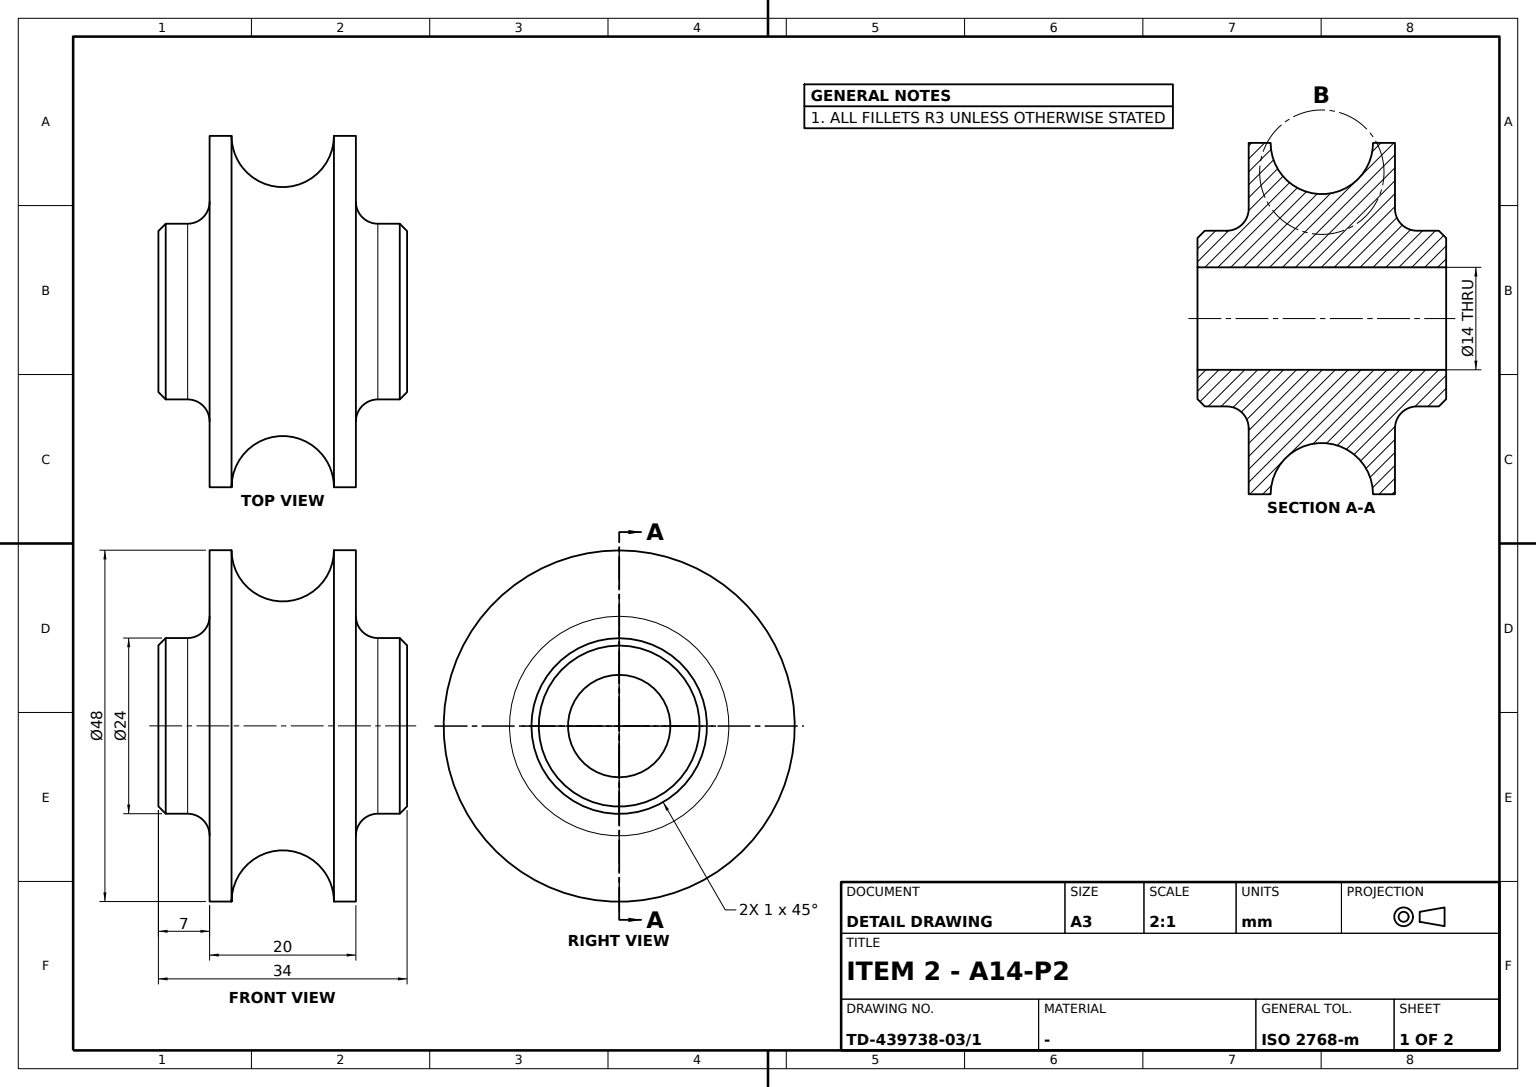
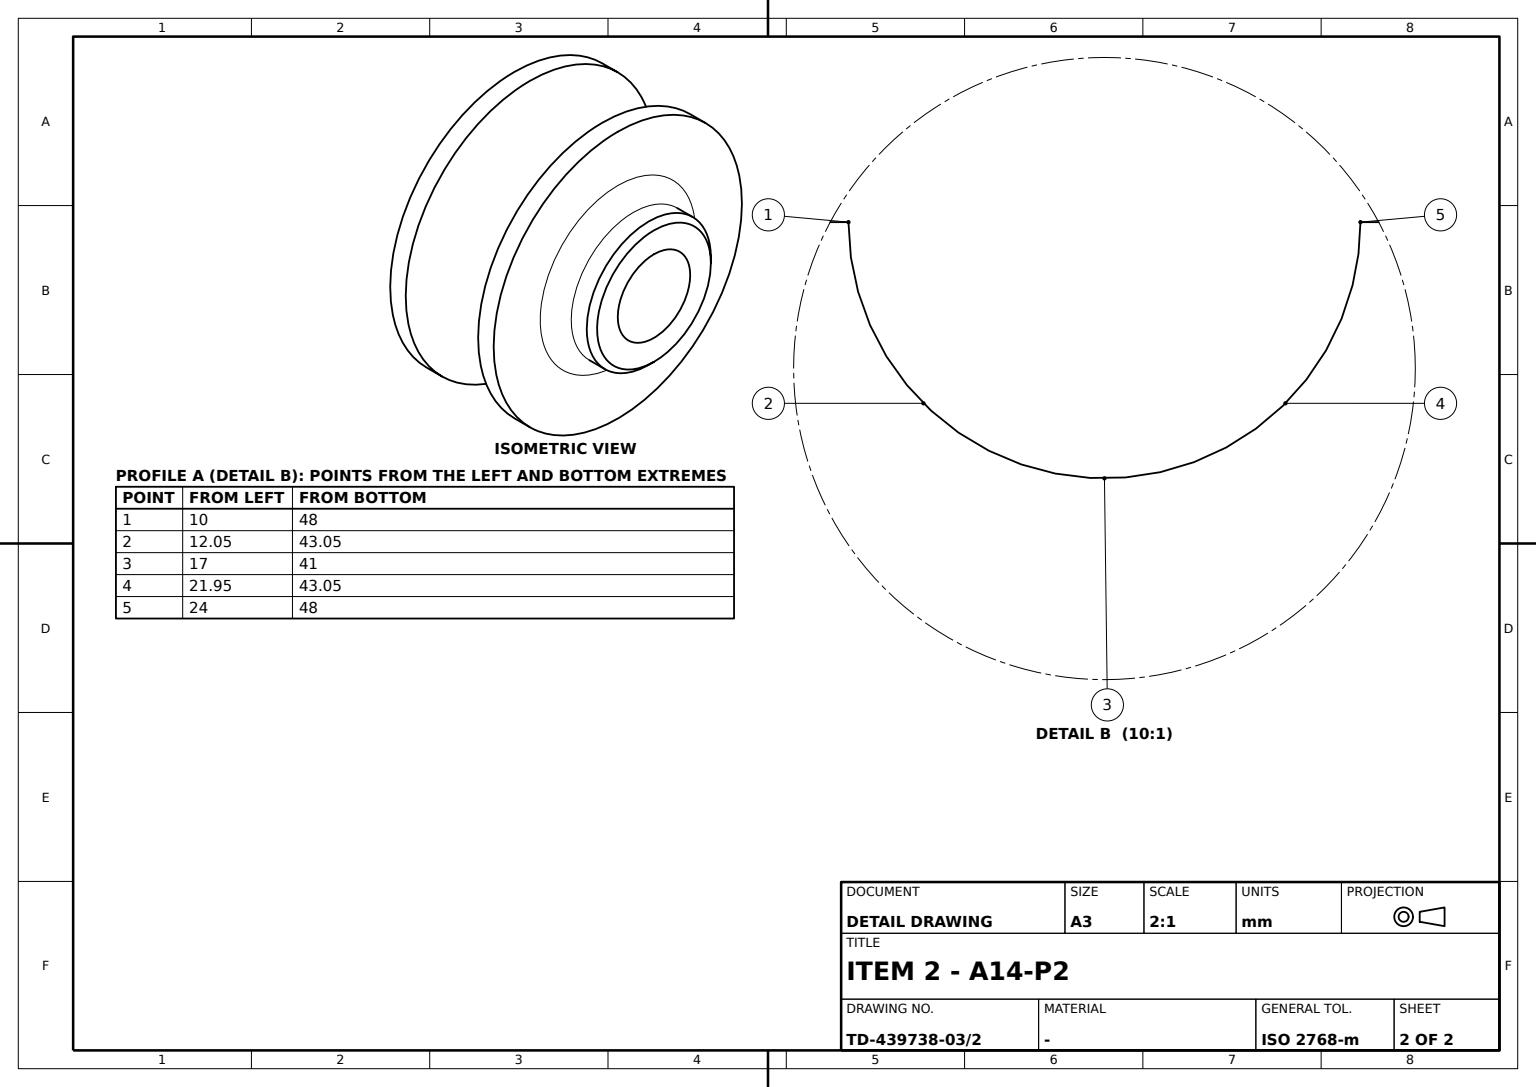
ISO-10303-21;
HEADER;
FILE_DESCRIPTION((''),'2;1');
FILE_NAME('','',(''),(''),'','','');
FILE_SCHEMA(('AUTOMOTIVE_DESIGN'));
ENDSEC;
DATA;
#1=APPLICATION_CONTEXT('');
#2=PRODUCT_CONTEXT('',#1,'mechanical');
#3=PRODUCT('','','',(#2));
#4=PRODUCT_DEFINITION_FORMATION('','',#3);
#5=PRODUCT_DEFINITION_CONTEXT('',#1,'design');
#6=PRODUCT_DEFINITION('','',#4,#5);
#7=PRODUCT_DEFINITION_SHAPE('','',#6);
#8=(LENGTH_UNIT()NAMED_UNIT(*)SI_UNIT(.MILLI.,.METRE.));
#9=(NAMED_UNIT(*)PLANE_ANGLE_UNIT()SI_UNIT($,.RADIAN.));
#10=(NAMED_UNIT(*)SI_UNIT($,.STERADIAN.)SOLID_ANGLE_UNIT());
#11=UNCERTAINTY_MEASURE_WITH_UNIT(LENGTH_MEASURE(0.005),#8,'distance_accuracy_value','');
#12=(GEOMETRIC_REPRESENTATION_CONTEXT(3)GLOBAL_UNCERTAINTY_ASSIGNED_CONTEXT((#11))GLOBAL_UNIT_ASSIGNED_CONTEXT((#8,#9,#10))REPRESENTATION_CONTEXT('',''));
#13=CARTESIAN_POINT('',(-16.,12.,0.));
#14=VERTEX_POINT('',#13);
#15=CARTESIAN_POINT('',(-16.,0.,0.));
#16=DIRECTION('',(1.,0.,0.));
#17=DIRECTION('',(0.,1.,0.));
#18=AXIS2_PLACEMENT_3D('',#15,#16,#17);
#19=CIRCLE('',#18,12.);
#20=EDGE_CURVE('',#14,#14,#19,.F.);
#21=ORIENTED_EDGE('',*,*,#20,.F.);
#22=EDGE_LOOP('',(#21));
#23=FACE_BOUND('',#22,.T.);
#24=CARTESIAN_POINT('',(-13.,0.,12.));
#25=VERTEX_POINT('',#24);
#26=CARTESIAN_POINT('',(-13.,0.,0.));
#27=DIRECTION('',(-1.,0.,0.));
#28=DIRECTION('',(0.,0.,1.));
#29=AXIS2_PLACEMENT_3D('',#26,#27,#28);
#30=CIRCLE('',#29,12.);
#31=EDGE_CURVE('',#25,#25,#30,.T.);
#32=ORIENTED_EDGE('',*,*,#31,.T.);
#33=EDGE_LOOP('',(#32));
#34=FACE_BOUND('',#33,.T.);
#35=CARTESIAN_POINT('',(0.,0.,0.));
#36=AXIS2_PLACEMENT_3D('',#35,#27,#17);
#37=CYLINDRICAL_SURFACE('',#36,12.);
#38=ADVANCED_FACE('',(#23,#34),#37,.T.);
#39=CARTESIAN_POINT('',(13.,0.,12.));
#40=VERTEX_POINT('',#39);
#41=CARTESIAN_POINT('',(13.,0.,0.));
#42=AXIS2_PLACEMENT_3D('',#41,#27,#28);
#43=CIRCLE('',#42,12.);
#44=EDGE_CURVE('',#40,#40,#43,.T.);
#45=ORIENTED_EDGE('',*,*,#44,.F.);
#46=EDGE_LOOP('',(#45));
#47=FACE_BOUND('',#46,.T.);
#48=CARTESIAN_POINT('',(16.,-12.,0.));
#49=VERTEX_POINT('',#48);
#50=CARTESIAN_POINT('',(16.,0.,0.));
#51=DIRECTION('',(0.,-1.,0.));
#52=AXIS2_PLACEMENT_3D('',#50,#27,#51);
#53=CIRCLE('',#52,12.);
#54=EDGE_CURVE('',#49,#49,#53,.T.);
#55=ORIENTED_EDGE('',*,*,#54,.T.);
#56=EDGE_LOOP('',(#55));
#57=FACE_BOUND('',#56,.T.);
#58=ADVANCED_FACE('',(#47,#57),#37,.T.);
#59=CARTESIAN_POINT('',(17.,0.,7.));
#60=VERTEX_POINT('',#59);
#61=CARTESIAN_POINT('',(17.,0.,0.));
#62=AXIS2_PLACEMENT_3D('',#61,#27,#28);
#63=CIRCLE('',#62,7.);
#64=EDGE_CURVE('',#60,#60,#63,.F.);
#65=ORIENTED_EDGE('',*,*,#64,.F.);
#66=EDGE_LOOP('',(#65));
#67=FACE_BOUND('',#66,.T.);
#68=CARTESIAN_POINT('',(17.,0.,11.));
#69=VERTEX_POINT('',#68);
#70=CIRCLE('',#62,11.);
#71=EDGE_CURVE('',#69,#69,#70,.T.);
#72=ORIENTED_EDGE('',*,*,#71,.F.);
#73=EDGE_LOOP('',(#72));
#74=FACE_BOUND('',#73,.T.);
#75=AXIS2_PLACEMENT_3D('',#61,#27,#17);
#76=PLANE('',#75);
#77=ADVANCED_FACE('',(#67,#74),#76,.F.);
#78=CARTESIAN_POINT('',(-10.,0.,24.));
#79=VERTEX_POINT('',#78);
#80=CARTESIAN_POINT('',(-10.,0.,0.));
#81=AXIS2_PLACEMENT_3D('',#80,#27,#28);
#82=CIRCLE('',#81,24.);
#83=EDGE_CURVE('',#79,#79,#82,.T.);
#84=ORIENTED_EDGE('',*,*,#83,.T.);
#85=EDGE_LOOP('',(#84));
#86=FACE_BOUND('',#85,.T.);
#87=CARTESIAN_POINT('',(-10.,0.,15.));
#88=VERTEX_POINT('',#87);
#89=CIRCLE('',#81,15.);
#90=EDGE_CURVE('',#88,#88,#89,.T.);
#91=ORIENTED_EDGE('',*,*,#90,.F.);
#92=EDGE_LOOP('',(#91));
#93=FACE_BOUND('',#92,.T.);
#94=AXIS2_PLACEMENT_3D('',#78,#27,#17);
#95=PLANE('',#94);
#96=ADVANCED_FACE('',(#86,#93),#95,.T.);
#97=CARTESIAN_POINT('',(7.,0.,24.));
#98=VERTEX_POINT('',#97);
#99=CARTESIAN_POINT('',(7.,0.,0.));
#100=AXIS2_PLACEMENT_3D('',#99,#27,#28);
#101=CIRCLE('',#100,24.);
#102=EDGE_CURVE('',#98,#98,#101,.T.);
#103=ORIENTED_EDGE('',*,*,#102,.T.);
#104=EDGE_LOOP('',(#103));
#105=FACE_BOUND('',#104,.T.);
#106=CARTESIAN_POINT('',(-7.,0.,24.));
#107=VERTEX_POINT('',#106);
#108=CARTESIAN_POINT('',(-7.,0.,0.));
#109=AXIS2_PLACEMENT_3D('',#108,#27,#28);
#110=CIRCLE('',#109,24.);
#111=EDGE_CURVE('',#107,#107,#110,.T.);
#112=ORIENTED_EDGE('',*,*,#111,.F.);
#113=EDGE_LOOP('',(#112));
#114=FACE_BOUND('',#113,.T.);
#115=TOROIDAL_SURFACE('',#36,24.,7.);
#116=ADVANCED_FACE('',(#105,#114),#115,.F.);
#117=ORIENTED_EDGE('',*,*,#90,.T.);
#118=EDGE_LOOP('',(#117));
#119=FACE_BOUND('',#118,.T.);
#120=ORIENTED_EDGE('',*,*,#31,.F.);
#121=EDGE_LOOP('',(#120));
#122=FACE_BOUND('',#121,.T.);
#123=DIRECTION('',(0.,-0.023596585,0.999721562));
#124=AXIS2_PLACEMENT_3D('',#26,#27,#123);
#125=TOROIDAL_SURFACE('',#124,15.,3.);
#126=ADVANCED_FACE('',(#119,#122),#125,.F.);
#127=ORIENTED_EDGE('',*,*,#44,.T.);
#128=EDGE_LOOP('',(#127));
#129=FACE_BOUND('',#128,.T.);
#130=CARTESIAN_POINT('',(10.,0.,15.));
#131=VERTEX_POINT('',#130);
#132=CARTESIAN_POINT('',(10.,0.,0.));
#133=AXIS2_PLACEMENT_3D('',#132,#27,#28);
#134=CIRCLE('',#133,15.);
#135=EDGE_CURVE('',#131,#131,#134,.T.);
#136=ORIENTED_EDGE('',*,*,#135,.F.);
#137=EDGE_LOOP('',(#136));
#138=FACE_BOUND('',#137,.T.);
#139=AXIS2_PLACEMENT_3D('',#41,#27,#123);
#140=TOROIDAL_SURFACE('',#139,15.,3.);
#141=ADVANCED_FACE('',(#129,#138),#140,.F.);
#142=ORIENTED_EDGE('',*,*,#64,.T.);
#143=EDGE_LOOP('',(#142));
#144=FACE_BOUND('',#143,.T.);
#145=CARTESIAN_POINT('',(-17.,0.,7.));
#146=VERTEX_POINT('',#145);
#147=CARTESIAN_POINT('',(-17.,0.,0.));
#148=AXIS2_PLACEMENT_3D('',#147,#27,#28);
#149=CIRCLE('',#148,7.);
#150=EDGE_CURVE('',#146,#146,#149,.T.);
#151=ORIENTED_EDGE('',*,*,#150,.T.);
#152=EDGE_LOOP('',(#151));
#153=FACE_BOUND('',#152,.T.);
#154=CARTESIAN_POINT('',(-4.5,0.,0.));
#155=AXIS2_PLACEMENT_3D('',#154,#16,#17);
#156=CYLINDRICAL_SURFACE('',#155,7.);
#157=ADVANCED_FACE('',(#144,#153),#156,.F.);
#158=CARTESIAN_POINT('',(-17.,0.,11.));
#159=VERTEX_POINT('',#158);
#160=CIRCLE('',#148,11.);
#161=EDGE_CURVE('',#159,#159,#160,.T.);
#162=ORIENTED_EDGE('',*,*,#161,.T.);
#163=EDGE_LOOP('',(#162));
#164=FACE_BOUND('',#163,.T.);
#165=ORIENTED_EDGE('',*,*,#150,.F.);
#166=EDGE_LOOP('',(#165));
#167=FACE_BOUND('',#166,.T.);
#168=CARTESIAN_POINT('',(-17.,0.,12.));
#169=AXIS2_PLACEMENT_3D('',#168,#27,#17);
#170=PLANE('',#169);
#171=ADVANCED_FACE('',(#164,#167),#170,.T.);
#172=ORIENTED_EDGE('',*,*,#135,.T.);
#173=EDGE_LOOP('',(#172));
#174=FACE_BOUND('',#173,.T.);
#175=CARTESIAN_POINT('',(10.,0.,24.));
#176=VERTEX_POINT('',#175);
#177=CIRCLE('',#133,24.);
#178=EDGE_CURVE('',#176,#176,#177,.T.);
#179=ORIENTED_EDGE('',*,*,#178,.F.);
#180=EDGE_LOOP('',(#179));
#181=FACE_BOUND('',#180,.T.);
#182=CARTESIAN_POINT('',(10.,0.,12.));
#183=AXIS2_PLACEMENT_3D('',#182,#27,#17);
#184=PLANE('',#183);
#185=ADVANCED_FACE('',(#174,#181),#184,.F.);
#186=ORIENTED_EDGE('',*,*,#102,.F.);
#187=EDGE_LOOP('',(#186));
#188=FACE_BOUND('',#187,.T.);
#189=ORIENTED_EDGE('',*,*,#178,.T.);
#190=EDGE_LOOP('',(#189));
#191=FACE_BOUND('',#190,.T.);
#192=CYLINDRICAL_SURFACE('',#36,24.);
#193=ADVANCED_FACE('',(#188,#191),#192,.T.);
#194=ORIENTED_EDGE('',*,*,#83,.F.);
#195=EDGE_LOOP('',(#194));
#196=FACE_BOUND('',#195,.T.);
#197=ORIENTED_EDGE('',*,*,#111,.T.);
#198=EDGE_LOOP('',(#197));
#199=FACE_BOUND('',#198,.T.);
#200=ADVANCED_FACE('',(#196,#199),#192,.T.);
#201=ORIENTED_EDGE('',*,*,#54,.F.);
#202=EDGE_LOOP('',(#201));
#203=FACE_BOUND('',#202,.T.);
#204=ORIENTED_EDGE('',*,*,#71,.T.);
#205=EDGE_LOOP('',(#204));
#206=FACE_BOUND('',#205,.T.);
#207=CARTESIAN_POINT('',(28.,0.,0.));
#208=DIRECTION('',(0.,0.520296023,-0.853985977));
#209=AXIS2_PLACEMENT_3D('',#207,#27,#208);
#210=CONICAL_SURFACE('',#209,0.,0.785398163);
#211=ADVANCED_FACE('',(#203,#206),#210,.T.);
#212=ORIENTED_EDGE('',*,*,#161,.F.);
#213=EDGE_LOOP('',(#212));
#214=FACE_BOUND('',#213,.T.);
#215=ORIENTED_EDGE('',*,*,#20,.T.);
#216=EDGE_LOOP('',(#215));
#217=FACE_BOUND('',#216,.T.);
#218=CARTESIAN_POINT('',(-28.,0.,0.));
#219=DIRECTION('',(0.,-0.520296023,0.853985977));
#220=AXIS2_PLACEMENT_3D('',#218,#16,#219);
#221=CONICAL_SURFACE('',#220,0.,0.785398163);
#222=ADVANCED_FACE('',(#214,#217),#221,.T.);
#223=CLOSED_SHELL('',(#38,#58,#77,#96,#116,#126,#141,#157,#171,#185,#193,#200,#211,#222));
#224=MANIFOLD_SOLID_BREP('',#223);
#225=ADVANCED_BREP_SHAPE_REPRESENTATION('',(#224),#12);
#226=SHAPE_DEFINITION_REPRESENTATION(#7,#225);
ENDSEC;
END-ISO-10303-21;
